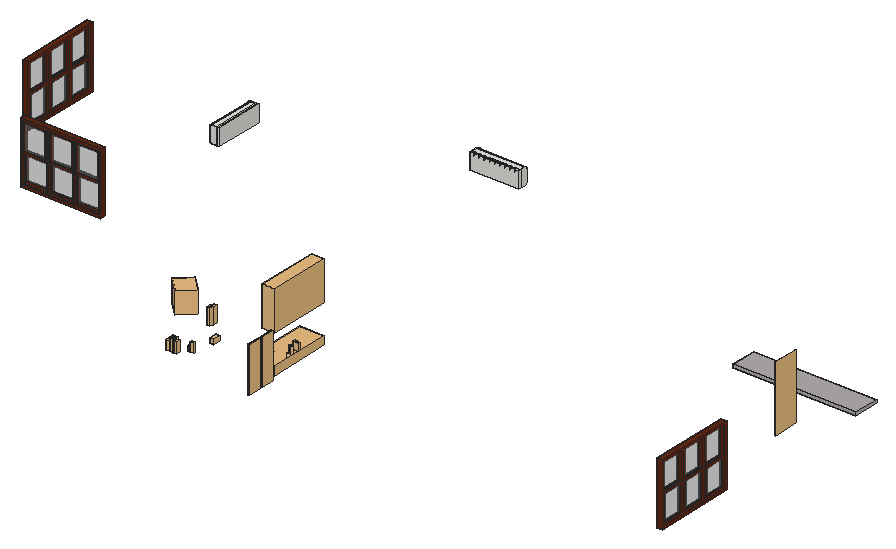
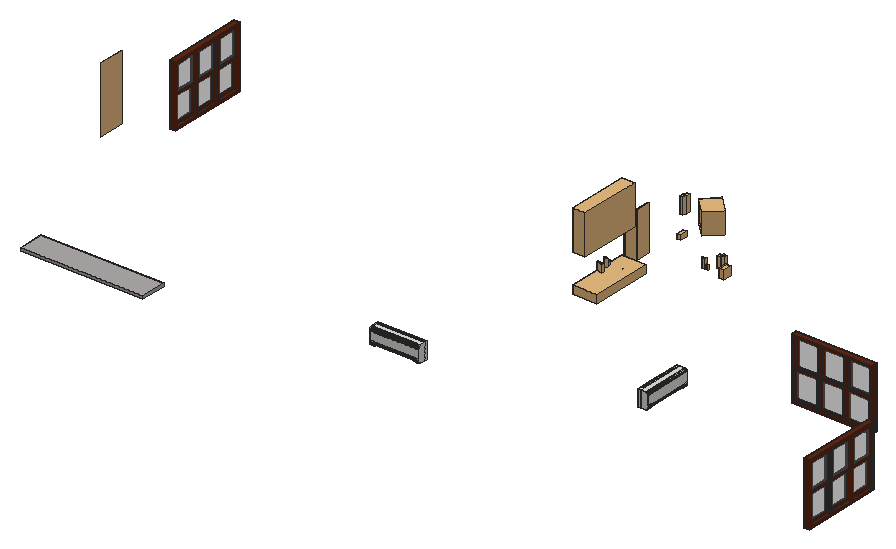
# SketchUp Ruby script. Lengths in inches.
U = 1.inch
M = Sketchup.active_model
def pt(a) = Geom::Point3d.new(a.map { |v| v * U })
def face(e, loops, mat)
  f = e.add_face(loops[0].map { |a| pt(a) })
  loops[1..].each { |l| e.add_face(l.map { |a| pt(a) }).erase! }
  f.material = f.back_material = mat if mat
  f
end
# faces: each face lists its corners as indices into pts; further lists are holes
def faces(e, pts, list, mat = nil) = list.each { |f| face(e, (f[0].is_a?(Array) ? f : [f]).map { |l| l.map { |i| pts[i] } }, mat) }
# xy, xz, yz: faces in a plane at the given z, y or x. An outline is a flat list of corners, or four numbers for a rectangle; further outlines are holes
def ring(l) = l.size == 4 ? [[l[0], l[1]], [l[2], l[1]], [l[2], l[3]], [l[0], l[3]]] : l.each_slice(2).to_a
def flat(e, list, mat, &to3) = list.each { |f| face(e, (f[0].is_a?(Array) ? f : [f]).map { |l| ring(l).map { |u, v| to3.(u, v) } }, mat) }
def xy(e, z, list, mat = nil) = flat(e, list, mat) { |x, y| [x, y, z] }
def xz(e, y, list, mat = nil) = flat(e, list, mat) { |x, z| [x, y, z] }
def yz(e, x, list, mat = nil) = flat(e, list, mat) { |y, z| [x, y, z] }
def lines(e, pts, list) = list.each { |a, b| e.add_line(pt(pts[a]), pt(pts[b])) }
# prism: a flat outline (further loops are holes) pulled along v
def prism(e, loops, v, mat = nil)
  f = face(e, loops, mat); d = Geom::Vector3d.new(v.map { |x| x * U })
  f.pushpull(f.normal.samedirection?(d) ? d.length : -d.length)
end
def box(e, o, s, mat = nil) = prism(e, [[o, [o[0] + s[0], o[1], o[2]], [o[0] + s[0], o[1] + s[1], o[2]], [o[0], o[1] + s[1], o[2]]]], [0, 0, s[2]], mat)
def at(x, y, z, deg = 0) = Geom::Transformation.translation(pt([x, y, z])) * Geom::Transformation.rotation(ORIGIN, Z_AXIS, deg.degrees)
def axes(o, x, y, z) = Geom::Transformation.new([*x, 0, *y, 0, *z, 0, *pt(o).to_a, 1])
def part(name) = M.definitions.add(name)
# library, detail: a bought-in or finely detailed component or shape, given as its bounding box
def library(name, o, s) = part(name).tap { |d| box(d.entities, o, s) }
def detail(e, o, s) = box(e.add_group.entities, o, s)
def put(e, d, t, mat = nil) = e.add_instance(d, t).tap { |i| i.material = mat if mat }
def group(e, t, mat = nil) = e.add_group.tap { |g| g.transformation = t; g.material = mat if mat }.entities
root = M.entities
M.materials.add("[0084_MediumTurquoise]").color = [178, 172, 172]
M.materials.add("[Color_004]").color = [142, 142, 142]
M.materials.add("[Color_005]").color = [114, 114, 114]
M.materials.add("[Color_007]").color = [58, 58, 58]
M.materials.add("[Color_B17]").color = [102, 40, 20]
M.materials.add("[Color_C12]").color = [153, 91, 30]
M.materials.add("[Translucent_Glass_Gray]").color = [128, 128, 128]
M.materials["[Translucent_Glass_Gray]"].alpha = 0.5
c1 = library("Group\#168",[0,0,0],[3.19,4.75,5.75])
c2 = library("Group\#184",[0,0,0],[13.47,43.07,1.47])
c3 = library("ear swab",[42.94,49.125,-0.01],[11.74,6.52,7.19])
c4 = library("Group\#182",[-0.16,-0.23,0],[24.67,28.96,29.58])
c5 = library("Group\#176",[0,0,0],[6.09,14.19,2.01])
c6 = library("Group\#177",[0,0,0],[5.65,13.74,2.92])
c7 = library("Group\#180",[0,0,0],[21.92,21.92,23.47])
c8 = library("Group\#181",[0,0,0],[23.26,37.79,80.08])
c9 = part("Framed panel")
g1 = group(c9.entities,at(0,0,0))
prism(g1,[[[0,22.64,0],[21.26,22.64,0],[21.26,0,0],[0,0,0]],[[1.57,1.57,0],[19.69,1.57,0],[19.69,21.0625,0],[1.57,21.0625,0]]],[0,0,1.57],"[Color_B17]")
g2 = group(c9.entities,at(1.57,1.57,1.02))
xy(g2,0,[[0,0,18.11,19.49]],"[Translucent_Glass_Gray]")
c10 = part("Group\#25")
put(c10.entities,c9,at(0,21.0625,1.57))
put(c10.entities,c9,at(0,0,0))
c11 = part("Group\#47")
g3 = group(c11.entities,at(0,0,0))
prism(g3,[[[70.87,0,0],[0,0,0],[0,47.24,0],[70.87,47.24,0]],[[47.83,1.77,0],[69.09,1.77,0],[69.09,45.47,0],[47.83,45.47,0]],[[46.0625,45.47,0],[24.8,45.47,0],[24.8,1.77,0],[46.0625,1.77,0]],[[1.77,1.77,0],[23.03,1.77,0],[23.03,45.47,0],[1.77,45.47,0]]],[0,0,4.33],"[Color_B17]")
put(c11.entities,c10,at(1.77,1.77,0.59))
put(c11.entities,c10,at(24.8,1.77,0.59))
put(c11.entities,c10,at(47.83,1.77,0.59))
c12 = part("Group\#165")
xy(c12.entities,0,[[3.14,0.77,2.7,0.83,2.28,1,1.93,1.27,1.65,1.63,1.48,2.04,4.8,2.93,4.86,2.49,4.8,2.04,4.63,1.63,4.36,1.27,4,1,3.59,0.83],[24.03,0.77,23.59,0.83,23.17,1,22.81,1.27,22.54,1.63,25.25,3.7,25.52,3.35,25.69,2.93,25.75,2.49,25.69,2.04,25.52,1.63,25.25,1.27,24.89,1,24.48,0.83],[22.54,1.63,22.37,2.04,22.3125,2.49,22.37,2.93,22.54,3.35,22.81,3.7,23.17,3.98,23.59,4.15,24.03,4.21,24.48,4.15,24.89,3.98,25.25,3.7],[1.48,2.04,1.42,2.49,1.48,2.93,1.65,3.35,1.93,3.7,2.28,3.98,2.7,4.15,3.14,4.21,3.59,4.15,4,3.98,4.36,3.7,4.63,3.35,4.8,2.93]],"[Color_005]")
xy(c12.entities,2.2,[[3.14,0.77,3.59,0.83,4,1,4.36,1.27,4.63,1.63,4.8,2.04,4.86,2.49,4.8,2.93,4.63,3.35,4.36,3.7,4,3.98,3.59,4.15,3.14,4.21,2.7,4.15,2.28,3.98,1.93,3.7,1.65,3.35,1.48,2.93,1.42,2.49,1.48,2.04,1.65,1.63,1.93,1.27,2.28,1,2.7,0.83],[24.03,0.77,24.48,0.83,24.89,1,25.25,1.27,25.52,1.63,25.69,2.04,25.75,2.49,25.69,2.93,25.52,3.35,25.25,3.7,24.89,3.98,24.48,4.15,24.03,4.21,23.59,4.15,23.17,3.98,22.81,3.7,22.54,3.35,22.37,2.93,22.3125,2.49,22.37,2.04,22.54,1.63,22.81,1.27,23.17,1,23.59,0.83]])
p = [[2.28,1,0],[2.7,0.83,0],[2.7,0.83,2.2],[2.28,1,2.2],[3.14,0.77,0],[3.14,0.77,2.2],
  [3.59,0.83,0],[3.59,0.83,2.2],[4,1,0],[4,1,2.2],[23.17,1,0],[23.59,0.83,0],
  [23.59,0.83,2.2],[23.17,1,2.2],[24.03,0.77,0],[24.03,0.77,2.2],[24.48,0.83,0],[24.48,0.83,2.2],
  [24.89,1,0],[24.89,1,2.2],[1.93,1.27,0],[1.93,1.27,2.2],[4.36,1.27,0],[4.36,1.27,2.2],
  [22.81,1.27,0],[22.81,1.27,2.2],[25.25,1.27,0],[25.25,1.27,2.2],[1.65,1.63,0],[1.65,1.63,2.2],
  [4.63,1.63,0],[4.63,1.63,2.2],[22.54,1.63,0],[22.54,1.63,2.2],[25.52,1.63,0],[25.52,1.63,2.2],
  [1.48,2.04,0],[1.48,2.04,2.2],[4.8,2.04,0],[4.8,2.04,2.2],[22.37,2.04,0],[22.37,2.04,2.2],
  [25.69,2.04,0],[25.69,2.04,2.2],[1.42,2.49,0],[1.42,2.49,2.2],[4.86,2.49,0],[4.86,2.49,2.2],
  [22.3125,2.49,0],[22.3125,2.49,2.2],[25.75,2.49,0],[25.75,2.49,2.2],[1.48,2.93,0],[1.48,2.93,2.2],
  [4.8,2.93,0],[4.8,2.93,2.2],[22.37,2.93,0],[22.37,2.93,2.2],[25.69,2.93,0],[25.69,2.93,2.2],
  [1.65,3.35,0],[1.65,3.35,2.2],[4.63,3.35,0],[4.63,3.35,2.2],[22.54,3.35,0],[22.54,3.35,2.2],
  [25.52,3.35,0],[25.52,3.35,2.2],[1.93,3.7,0],[1.93,3.7,2.2],[4.36,3.7,0],[4.36,3.7,2.2],
  [22.81,3.7,0],[22.81,3.7,2.2],[25.25,3.7,0],[25.25,3.7,2.2],[2.28,3.98,0],[2.28,3.98,2.2],
  [4,3.98,0],[4,3.98,2.2],[23.17,3.98,0],[23.17,3.98,2.2],[24.89,3.98,0],[24.89,3.98,2.2],
  [2.7,4.15,0],[2.7,4.15,2.2],[3.59,4.15,0],[3.59,4.15,2.2],[23.59,4.15,0],[23.59,4.15,2.2],
  [24.48,4.15,0],[24.48,4.15,2.2],[3.14,4.21,0],[3.14,4.21,2.2],[24.03,4.21,0],[24.03,4.21,2.2]]
faces(c12.entities,p,[[0,1,2,3],[1,4,5,2],[4,6,7,5],[6,8,9,7],[10,11,12,13],[11,14,15,12],[14,16,17,15],[16,18,19,17],
  [20,0,3,21],[8,22,23,9],[24,10,13,25],[18,26,27,19],[28,20,21,29],[22,30,31,23],[32,24,25,33],[26,34,35,27],
  [36,28,29,37],[30,38,39,31],[40,32,33,41],[34,42,43,35],[44,36,37,45],[38,46,47,39],[48,40,41,49],[42,50,51,43],
  [52,44,45,53],[46,54,55,47],[56,48,49,57],[50,58,59,51],[60,52,53,61],[54,62,63,55],[64,56,57,65],[58,66,67,59],
  [68,60,61,69],[62,70,71,63],[72,64,65,73],[66,74,75,67],[76,68,69,77],[70,78,79,71],[80,72,73,81],[74,82,83,75],
  [84,76,77,85],[78,86,87,79],[88,80,81,89],[82,90,91,83],[92,84,85,93],[86,92,93,87],[94,88,89,95],[90,94,95,91]],"[Color_005]")
g4 = group(c12.entities,at(0,0,1.83),"[Color_005]")
box(g4,[0,0,0],[27.7,4.93,1.59])
c13 = library("Group\#189",[-0.38,0,0],[4.27,10.97,14.2])
c14 = library("Group\#188",[0,0,0],[19.07,47.48,6.54])
c15 = library("Group\#186",[0,0,0],[47.48,30.74,9.84])
c16 = library("Group\#224",[0,202.4,-2.65],[190.5,180.61,2.65])
c17 = library("Group\#73",[-80.34,-149.03,-93.91],[1.18,2.79,3])
c18 = library("Group\#74",[-80.34,-139.83,-93.89],[1.18,2.84,2.98])
c19 = library("Group\#63",[-80.46,-65.36,-92.6],[1.38,3.58,3.59])
p = [[1618.6875,177.45,34.42],[1618.76,177.12,35.41],[1618.76,177.1,35.41]]
faces(root,p,[[0,1,2]])
g5 = group(root,at(1599.51,140.375,64.56))
detail(g5,[-0.37,-2.82,0],[2.54,2.53,12.33])
g6 = group(root,at(1571.03,141.11,35.64))
detail(g6,[-1.27,-3.0625,0],[2.54,2.53,9.2])
g7 = group(root,at(1575.59,140.06,35.64))
detail(g7,[-3,-1.73,0],[2.54,2.53,8.61])
g8 = group(root,at(1602.34,143.09,64.56))
detail(g8,[-2.7,-2.7,0],[2.7,2.7,12.33])
put(root,c1,axes([1568.21,147.6,33.83],[-1.2,0,0],[0,-1.416,0],[0,0,1.2]))
put(root,c2,axes([1630.57,149.66,26.11],[0,-0.77,0],[0,0,0.80496],[-1,0,0]))
put(root,c3,axes([1625.67,120.32,49.79],[0,0.5,0],[-0.5,0,0],[0,0,0.5]))
put(root,c4,axes([1574.96,155.51,64.56],[-0.39598,-0.39598,0],[0.39598,-0.39598,0],[0,0,0.56]))
put(root,c5,axes([1579.89,146.53,35.64],[0.5,0,0],[0,0,0.5],[0,-0.5,0]))
put(root,c6,axes([1578.03,146.54,35.64],[0.25,0,0],[0,0,0.25],[0,-0.25,0]))
put(root,c2,axes([1630.57,162.07,26.11],[0,-0.77,0],[0,0,0.80496],[-1,0,0]))
put(root,c7,axes([1628.03,178.13,35.52],[0.06654,-0.06654,0],[0.06654,0.06654,0],[0,0,0.09411]))
put(root,c8,axes([1628.3125,182.5,35.43],[-0.03711,-0.06428,0],[0.06428,-0.03711,0],[0,0,0.07422]))
put(root,c11,axes([1939.4375,213.95,36],[0,-0.87489,0],[0,0,1.016],[-1,0,0]))
put(root,c12,axes([1618.76,192.77,24.02],[0,-0.3762,0],[0,0,0.25582],[-0.3762,0,0]))
put(root,c13,axes([1626.17,188.26,35.43],[0,-0.39,0],[0.39,0,0],[0,0,0.39]),"[Color_005]")
put(root,c14,at(1630.57,211.45,28.89,-180))
put(root,c15,axes([1630.57,211.45,58.17],[0,-1,0],[0,0,1],[-1,0,0]))
put(root,c11,axes([1373.72,243.48,36],[0.87489,0,0],[0,0,1.016],[0,-1,0]))
put(root,c16,axes([1942.8125,275.9,0],[0,-0.10244,-0.00004],[0,-0.00011,0.28043],[-0.22,0,0]))
g9 = group(root,at(1470.58,328.97,79.75))
prism(g9,[[[-7.07,-15.5,-9.29],[-7.07,-15.45,-9.6],[-7.07,-15.52,-9.6],[-7.07,-15.57,-9.29]]],[0.1,0,0],"[Color_004]")
g10 = group(root,at(1470.58,328.97,79.75))
detail(g10,[-7.07,-15.51,-9.71],[0.1,0.08,0.08])
put(root,c17,axes([1470.58,328.97,79.75],[0.088,0,0],[0,0.10336,0],[0,0,0.10336]))
g11 = group(root,at(1470.58,328.97,79.75),"[Color_004]")
prism(g11,[[[-7.07,-15.07,-9.4],[-7.07,-14.96,-9.6],[-7.07,-14.92,-9.4],[-7.07,-14.85,-9.4],[-7.07,-14.91,-9.7],[-7.07,-14.98,-9.7],[-7.07,-15.15,-9.4]]],[0.1,0,0],"[Color_004]")
g12 = group(root,at(1470.58,328.97,79.75))
detail(g12,[-7.07,-14.86,-9.37],[0.1,0.08,0.08])
g13 = group(root,at(1470.58,328.97,79.75))
prism(g13,[[[-7.07,-14.79,-9.7],[-7.07,-14.84,-9.4],[-7.07,-14.77,-9.4],[-7.07,-14.72,-9.7]]],[0.1,0,0],"[Color_004]")
g14 = group(root,at(1470.58,328.97,79.75))
detail(g14,[-7.07,-14.73,-9.7],[0.1,0.25,0.41])
put(root,c18,axes([1470.58,328.97,79.75],[0.088,0,0],[0,0.10336,0],[0,0,0.10336]))
put(root,c19,axes([1470.57,328.97,79.75],[0.088,0,0],[0,0.10336,0],[0,0,0.10336]))
put(root,c11,axes([1334.35,357.95,36],[0,-0.87489,0],[0,0,1.016],[-1,0,0]))
g15 = group(root,at(1470.64,328.97,79.75))
xy(g15,-12.74,[[-1.73,-18.76,0,18.76]])
xy(g15,-2.26,[[-0.93,-15.67,-0.73,-11.93],[-0.64,-15.67,-0.43,-11.93],[-0.35,-15.67,-0.14,-11.93],[-0.93,-11.73,-0.73,-7.99],[-0.64,-11.73,-0.43,-7.99],
  [-0.35,-11.73,-0.14,-7.99],[-0.93,-7.79,-0.73,-4.04],[-0.64,-7.79,-0.43,-4.04],[-0.35,-7.79,-0.14,-4.04],[-0.93,-3.84,-0.73,-0.1],
  [-0.64,-3.84,-0.43,-0.1],[-0.35,-3.84,-0.14,-0.1],[-0.93,0.1,-0.73,3.84],[-0.64,0.1,-0.43,3.84],[-0.35,0.1,-0.14,3.84],
  [-0.93,4.04,-0.73,7.79],[-0.64,4.04,-0.43,7.79],[-0.35,4.04,-0.14,7.79],[-0.93,7.99,-0.73,11.73],[-0.64,7.99,-0.43,11.73],
  [-0.35,7.99,-0.14,11.73],[-0.93,11.93,-0.73,15.67],[-0.64,11.93,-0.43,15.67],[-0.35,11.93,-0.14,15.67]])
xy(g15,0,[[[-1.73,-18.76,0,18.76],[-0.93,4.04,-0.93,11.73,-0.73,11.73,-0.73,7.99,-0.93,7.99,-0.93,7.79,-0.73,7.79,-0.73,4.04],[-0.35,4.04,-0.35,7.79,-0.14,7.79,-0.14,7.99,-0.35,7.99,-0.35,11.73,-0.14,11.73,-0.14,4.04],[-0.64,11.93,-0.43,15.67],[-0.35,11.93,-0.14,15.67],[-0.93,11.93,-0.73,15.67],[-0.93,-15.67,-0.73,-11.93],[-0.35,-15.67,-0.14,-11.93],[-0.64,-15.67,-0.43,-11.93],[-0.64,4.04,-0.43,7.79],[-0.35,-7.79,-0.14,-4.04],[-0.64,-7.79,-0.43,-4.04],[-0.93,-7.79,-0.73,-4.04],[-0.64,7.99,-0.43,11.73],[-0.64,0.1,-0.43,3.84],[-0.35,0.1,-0.14,3.84],[-0.93,0.1,-0.73,3.84],[-0.35,-11.73,-0.14,-7.99],[-0.93,-11.73,-0.73,-7.99],[-0.93,-3.84,-0.73,-0.1],[-0.64,-3.84,-0.43,-0.1],[-0.35,-3.84,-0.14,-0.1],[-0.64,-11.73,-0.43,-7.99]]])
xz(g15,-18.76,[[-1.73,-12.74,0,0]])
xz(g15,-15.67,[[-0.93,-2.26,-0.73,0],[-0.64,-2.26,-0.43,0],[-0.35,-2.26,-0.14,0]])
xz(g15,-11.93,[[-0.93,-2.26,-0.73,0],[-0.64,-2.26,-0.43,0],[-0.35,-2.26,-0.14,0]])
xz(g15,-11.73,[[-0.93,-2.26,-0.73,0],[-0.64,-2.26,-0.43,0],[-0.35,-2.26,-0.14,0]])
xz(g15,-7.99,[[-0.93,-2.26,-0.73,0],[-0.64,-2.26,-0.43,0],[-0.35,-2.26,-0.14,0]])
xz(g15,-7.79,[[-0.93,-2.26,-0.73,0],[-0.64,-2.26,-0.43,0],[-0.35,-2.26,-0.14,0]])
xz(g15,-4.04,[[-0.93,-2.26,-0.73,0],[-0.64,-2.26,-0.43,0],[-0.35,-2.26,-0.14,0]])
xz(g15,-3.84,[[-0.93,-2.26,-0.73,0],[-0.64,-2.26,-0.43,0],[-0.35,-2.26,-0.14,0]])
xz(g15,-0.1,[[-0.93,-2.26,-0.73,0],[-0.64,-2.26,-0.43,0],[-0.35,-2.26,-0.14,0]])
xz(g15,0.1,[[-0.93,-2.26,-0.73,0],[-0.64,-2.26,-0.43,0],[-0.35,-2.26,-0.14,0]])
xz(g15,3.84,[[-0.93,-2.26,-0.73,0],[-0.64,-2.26,-0.43,0],[-0.35,-2.26,-0.14,0]])
xz(g15,4.04,[[-0.93,-2.26,-0.73,0],[-0.64,-2.26,-0.43,0],[-0.35,-2.26,-0.14,0]])
xz(g15,7.79,[[-0.93,-2.26,-0.73,0],[-0.64,-2.26,-0.43,0],[-0.35,-2.26,-0.14,0]])
xz(g15,7.99,[[-0.93,-2.26,-0.73,0],[-0.64,-2.26,-0.43,0],[-0.35,-2.26,-0.14,0]])
xz(g15,11.73,[[-0.93,-2.26,-0.73,0],[-0.64,-2.26,-0.43,0],[-0.35,-2.26,-0.14,0]])
xz(g15,11.93,[[-0.93,-2.26,-0.73,0],[-0.64,-2.26,-0.43,0],[-0.35,-2.26,-0.14,0]])
xz(g15,15.67,[[-0.93,-2.26,-0.73,0],[-0.64,-2.26,-0.43,0],[-0.35,-2.26,-0.14,0]])
xz(g15,18.76,[[-1.73,-12.74,0,0]])
yz(g15,-1.73,[[-18.76,-12.74,18.76,0]])
yz(g15,-0.93,[[-15.67,-2.26,-11.93,0],[-11.73,-2.26,-7.99,0],[-7.79,-2.26,-4.04,0],[-3.84,-2.26,-0.1,0],[0.1,-2.26,3.84,0],
  [4.04,-2.26,7.79,0],[7.99,-2.26,11.73,0],[11.93,-2.26,15.67,0]])
yz(g15,-0.73,[[-15.67,-2.26,-11.93,0],[-11.73,-2.26,-7.99,0],[-7.79,-2.26,-4.04,0],[-3.84,-2.26,-0.1,0],[0.1,-2.26,3.84,0],
  [4.04,-2.26,7.79,0],[7.99,-2.26,11.73,0],[11.93,-2.26,15.67,0]])
yz(g15,-0.64,[[-15.67,-2.26,-11.93,0],[-11.73,-2.26,-7.99,0],[-7.79,-2.26,-4.04,0],[-3.84,-2.26,-0.1,0],[0.1,-2.26,3.84,0],
  [4.04,-2.26,7.79,0],[7.99,-2.26,11.73,0],[11.93,-2.26,15.67,0]])
yz(g15,-0.43,[[-15.67,-2.26,-11.93,0],[-11.73,-2.26,-7.99,0],[-7.79,-2.26,-4.04,0],[-3.84,-2.26,-0.1,0],[0.1,-2.26,3.84,0],
  [4.04,-2.26,7.79,0],[7.99,-2.26,11.73,0],[11.93,-2.26,15.67,0]])
yz(g15,-0.35,[[-15.67,-2.26,-11.93,0],[-11.73,-2.26,-7.99,0],[-7.79,-2.26,-4.04,0],[-3.84,-2.26,-0.1,0],[0.1,-2.26,3.84,0],
  [4.04,-2.26,7.79,0],[7.99,-2.26,11.73,0],[11.93,-2.26,15.67,0]])
yz(g15,-0.14,[[-15.67,-2.26,-11.93,0],[-11.73,-2.26,-7.99,0],[-7.79,-2.26,-4.04,0],[-3.84,-2.26,-0.1,0],[0.1,-2.26,3.84,0],
  [4.04,-2.26,7.79,0],[7.99,-2.26,11.73,0],[11.93,-2.26,15.67,0]])
yz(g15,0,[[-18.76,-12.74,18.76,0]])
g16 = group(root,at(1470.64,328.97,79.75))
xy(g16,-12.74,[[-5.65,-18.76,-1.73,-15.875],[-5.65,15.875,-1.73,18.76]])
xy(g16,-9.91,[[-7.03,-15.875,-1.73,15.875]])
xy(g16,-9.7,[[-7.03,-3.48,-6.93,3.48]])
xy(g16,-9.07,[[-7.03,-3.48,-6.93,3.48]])
xy(g16,-8.96,[[-7.73,-18.76,-7.62,-15.875],[-7.62,-15.875,-7.03,15.875],[-7.73,15.875,-7.62,18.76]])
xy(g16,0,[[-5.65,-18.76,-1.73,18.76]])
xz(g16,-18.76,[[-5.65,-12.74,-1.73,-12.74,-1.73,0,-5.65,0,-5.65,-0.12,-5.96,-0.15,-6.26,-0.24,-6.54,-0.375,-6.81,-0.57,-7.04,-0.8,-7.24,-1.08,-7.41,-1.39,-7.53,-1.72,-7.6,-2.08,-7.62,-2.44,-7.62,-8.96,-7.73,-8.96,-7.73,-10.29,-7.7,-10.68,-7.625,-11.05,-7.5,-11.4,-7.33,-11.73,-7.12,-12.02,-6.87,-12.27,-6.59,-12.47,-6.29,-12.62,-5.97,-12.71]])
xz(g16,-15.875,[[-5.65,-12.74,-5.97,-12.71,-6.29,-12.62,-6.59,-12.47,-6.87,-12.27,-7.12,-12.02,-7.33,-11.73,-7.5,-11.4,-7.625,-11.05,-7.7,-10.68,-7.73,-10.29,-7.73,-8.96,-7.03,-8.96,-7.03,-9.91,-1.73,-9.91,-1.73,-12.74]])
xz(g16,-3.48,[[-7.03,-9.7,-6.93,-9.07]])
xz(g16,3.48,[[-7.03,-9.7,-6.93,-9.07]])
xz(g16,15.875,[[-5.65,-12.74,-1.73,-12.74,-1.73,-9.91,-7.03,-9.91,-7.03,-8.96,-7.73,-8.96,-7.73,-10.29,-7.7,-10.68,-7.625,-11.05,-7.5,-11.4,-7.33,-11.73,-7.12,-12.02,-6.87,-12.27,-6.59,-12.47,-6.29,-12.62,-5.97,-12.71]])
xz(g16,18.76,[[-5.65,-12.74,-5.97,-12.71,-6.29,-12.62,-6.59,-12.47,-6.87,-12.27,-7.12,-12.02,-7.33,-11.73,-7.5,-11.4,-7.625,-11.05,-7.7,-10.68,-7.73,-10.29,-7.73,-8.96,-7.62,-8.96,-7.62,-2.44,-7.6,-2.08,-7.53,-1.72,-7.41,-1.39,-7.24,-1.08,-7.04,-0.8,-6.81,-0.57,-6.54,-0.375,-6.26,-0.24,-5.96,-0.15,-5.65,-0.12,-5.65,0,-1.73,0,-1.73,-12.74]])
yz(g16,-7.73,[[-18.76,-10.29,-15.875,-8.96],[15.875,-10.29,18.76,-8.96]])
yz(g16,-7.62,[[-18.76,-8.96,18.76,-2.44]])
yz(g16,-7.03,[[[-15.875,-9.91,15.875,-8.96],[-3.48,-9.7,3.48,-9.07]]])
yz(g16,-6.93,[[-3.48,-9.7,3.48,-9.07]],"[Color_007]")
yz(g16,-5.65,[[-18.76,-0.12,18.76,0]])
yz(g16,-1.73,[[-18.76,-12.74,-15.875,-12.74,-15.875,-9.91,15.875,-9.91,15.875,-12.74,18.76,-12.74,18.76,0,-18.76,0]])
p = [[-6.29,-18.76,-12.62],[-6.29,-15.875,-12.62],[-5.97,-15.875,-12.71],[-5.97,-18.76,-12.71],[-5.65,-15.875,-12.74],[-5.65,-18.76,-12.74],
  [-6.29,15.875,-12.62],[-6.29,18.76,-12.62],[-5.97,18.76,-12.71],[-5.97,15.875,-12.71],[-5.65,18.76,-12.74],[-5.65,15.875,-12.74],
  [-6.59,-15.875,-12.47],[-6.59,-18.76,-12.47],[-6.59,15.875,-12.47],[-6.59,18.76,-12.47],[-6.87,-18.76,-12.27],[-6.87,-15.875,-12.27],
  [-6.87,15.875,-12.27],[-6.87,18.76,-12.27],[-7.12,-18.76,-12.02],[-7.12,-15.875,-12.02],[-7.12,15.875,-12.02],[-7.12,18.76,-12.02],
  [-7.33,-18.76,-11.73],[-7.33,-15.875,-11.73],[-7.33,15.875,-11.73],[-7.33,18.76,-11.73],[-7.5,-18.76,-11.4],[-7.5,-15.875,-11.4],
  [-7.5,15.875,-11.4],[-7.5,18.76,-11.4],[-7.625,-15.875,-11.05],[-7.625,-18.76,-11.05],[-7.625,15.875,-11.05],[-7.625,18.76,-11.05],
  [-7.7,-18.76,-10.68],[-7.7,-15.875,-10.68],[-7.7,15.875,-10.68],[-7.7,18.76,-10.68],[-7.73,-18.76,-10.29],[-7.73,-15.875,-10.29],
  [-7.73,15.875,-10.29],[-7.73,18.76,-10.29],[-7.62,18.76,-2.44],[-7.62,-18.76,-2.44],[-7.6,-18.76,-2.08],[-7.6,18.76,-2.08],
  [-7.53,-18.76,-1.72],[-7.53,18.76,-1.72],[-7.41,18.76,-1.39],[-7.41,-18.76,-1.39],[-7.24,-18.76,-1.08],[-7.24,18.76,-1.08],
  [-7.04,-18.76,-0.8],[-7.04,18.76,-0.8],[-6.81,-18.76,-0.57],[-6.81,18.76,-0.57],[-6.54,-18.76,-0.375],[-6.54,18.76,-0.375],
  [-6.26,18.76,-0.24],[-6.26,-18.76,-0.24],[-5.96,-18.76,-0.15],[-5.96,18.76,-0.15],[-5.65,-18.76,-0.12],[-5.65,18.76,-0.12]]
faces(g16,p,[[0,1,2,3],[4,5,3,2],[6,7,8,9],[10,11,9,8],[12,1,0,13],[6,14,15,7],[12,13,16,17],[15,14,18,19],
  [20,21,17,16],[22,23,19,18],[21,20,24,25],[23,22,26,27],[28,29,25,24],[30,31,27,26],[32,29,28,33],[30,34,35,31],
  [32,33,36,37],[35,34,38,39],[40,41,37,36],[42,43,39,38],[44,45,46,47],[48,49,47,46],[50,49,48,51],[50,51,52,53],
  [54,55,53,52],[55,54,56,57],[58,59,57,56],[60,59,58,61],[60,61,62,63],[64,65,63,62]])
g17 = group(root,at(1470.64,328.97,79.75))
prism(g17,[[[-7.73,18.74,-8.96],[-7.73,18.74,-2.44],[-7.7,18.74,-2.06],[-7.625,18.74,-1.6875],[-7.5,18.74,-1.33],[-7.33,18.74,-1.01],[-7.12,18.74,-0.72],[-6.87,18.74,-0.47],[-6.59,18.74,-0.27],[-6.29,18.74,-0.12],[-5.97,18.74,-0.03],[-5.65,18.74,0],[-5.65,18.74,-0.12],[-5.96,18.74,-0.15],[-6.26,18.74,-0.24],[-6.54,18.74,-0.375],[-6.81,18.74,-0.57],[-7.04,18.74,-0.8],[-7.24,18.74,-1.08],[-7.41,18.74,-1.39],[-7.53,18.74,-1.72],[-7.6,18.74,-2.08],[-7.62,18.74,-2.44],[-7.62,18.74,-8.96]]],[0,-37.47,0])
g18 = group(root,at(1470.64,328.97,79.75))
xy(g18,-12.375,[[-5.58,-15.875,-3.67,15.875]])
xy(g18,-10.42,[[-7.25,-15.875,-7,-9.1],[-7.25,-8.85,-7,4.71],[-7.25,4.95,-7,15.875]])
xy(g18,-9.91,[[-7,-15.875,-3.67,-15.875,-3.67,15.875,-7,15.875,-7,4.95,-7.25,4.95,-7.25,4.71,-7,4.71,-7,-8.85,-7.25,-8.85,-7.25,-9.1,-7,-9.1]])
xz(g18,-15.875,[[-5.58,-12.375,-3.67,-12.375,-3.67,-9.91,-7,-9.91,-7,-10.42,-7.25,-10.42,-7.24,-10.46,-7.23,-10.73,-7.17,-11.02,-7.07,-11.31,-6.93,-11.57,-6.76,-11.8,-6.5625,-12,-6.34,-12.16,-6.1,-12.28,-5.84,-12.35]])
xz(g18,-9.1,[[-7.25,-10.42,-7,-9.91]])
xz(g18,-8.85,[[-7.25,-10.42,-7,-9.91]])
xz(g18,4.71,[[-7.25,-10.42,-7,-9.91]])
xz(g18,4.95,[[-7.25,-10.42,-7,-9.91]])
xz(g18,15.875,[[-5.58,-12.375,-5.84,-12.35,-6.1,-12.28,-6.34,-12.16,-6.5625,-12,-6.76,-11.8,-6.93,-11.57,-7.07,-11.31,-7.17,-11.02,-7.23,-10.73,-7.24,-10.46,-7.25,-10.42,-7,-10.42,-7,-9.91,-3.67,-9.91,-3.67,-12.375]])
yz(g18,-7.25,[[-9.1,-10.42,-8.85,-9.91],[4.71,-10.42,4.95,-9.91]])
yz(g18,-7,[[-15.875,-10.42,-9.1,-9.91],[-8.85,-10.42,4.71,-9.91],[4.95,-10.42,15.875,-9.91]],"[Color_007]")
yz(g18,-3.67,[[-15.875,-12.375,15.875,-9.91]])
p = [[-5.58,15.875,-12.375],[-5.58,-15.875,-12.375],[-5.84,-15.875,-12.35],[-5.84,15.875,-12.35],[-6.34,15.875,-12.16],[-6.1,15.875,-12.28],
  [-6.1,-15.875,-12.28],[-6.34,-15.875,-12.16],[-6.5625,-15.875,-12],[-6.5625,15.875,-12],[-6.76,-15.875,-11.8],[-6.76,15.875,-11.8],
  [-6.93,-15.875,-11.57],[-6.93,15.875,-11.57],[-7.07,-15.875,-11.31],[-7.07,15.875,-11.31],[-7.17,15.875,-11.02],[-7.17,-15.875,-11.02],
  [-7.23,-15.875,-10.73],[-7.23,15.875,-10.73],[-7.24,-15.875,-10.46],[-7.24,-9.1,-10.46],[-7.24,-8.85,-10.46],[-7.24,4.71,-10.46],
  [-7.24,4.95,-10.46],[-7.24,15.875,-10.46],[-7.25,15.875,-10.42],[-7.25,-15.875,-10.42],[-7.25,-9.1,-10.42],[-7.25,-8.85,-10.42],
  [-7.25,4.71,-10.42],[-7.25,4.95,-10.42]]
faces(g18,p,[[0,1,2,3],[4,5,6,7],[6,5,3,2],[4,7,8,9],[10,11,9,8],[11,10,12,13],[14,15,13,12],[16,15,14,17],
  [16,17,18,19],[18,20,21,22,23,24,25,19]])
faces(g18,p,[[26,25,24,23,22,21,20,27,28,29,30,31]],"[Color_C12]")
g19 = group(root,at(1834.62,351.14,23.97),"[0084_MediumTurquoise]")
box(g19,[0,0,0],[94.73,19.71,2.36],"[0084_MediumTurquoise]")
g20 = group(root,at(1625.625,381.93,79.75))
xy(g20,-12.74,[[-18.76,0,18.76,1.73]])
xy(g20,-2.26,[[-15.67,0.14,-11.93,0.35],[-11.73,0.14,-7.99,0.35],[-7.79,0.14,-4.04,0.35],[-3.84,0.14,-0.1,0.35],[0.1,0.14,3.84,0.35],
  [4.04,0.14,7.79,0.35],[7.99,0.14,11.73,0.35],[11.93,0.14,15.67,0.35],[-15.67,0.43,-11.93,0.64],[-11.73,0.43,-7.99,0.64],
  [-7.79,0.43,-4.04,0.64],[-3.84,0.43,-0.1,0.64],[0.1,0.43,3.84,0.64],[4.04,0.43,7.79,0.64],[7.99,0.43,11.73,0.64],
  [11.93,0.43,15.67,0.64],[-15.67,0.73,-11.93,0.93],[-11.73,0.73,-7.99,0.93],[-7.79,0.73,-4.04,0.93],[-3.84,0.73,-0.1,0.93],
  [0.1,0.73,3.84,0.93],[4.04,0.73,7.79,0.93],[7.99,0.73,11.73,0.93],[11.93,0.73,15.67,0.93]])
xy(g20,0,[[[-18.76,0,18.76,1.73],[4.04,0.73,4.04,0.93,11.73,0.93,11.73,0.73,7.99,0.73,7.99,0.93,7.79,0.93,7.79,0.73],[4.04,0.14,4.04,0.35,7.79,0.35,7.79,0.14,7.99,0.14,7.99,0.35,11.73,0.35,11.73,0.14],[11.93,0.43,15.67,0.64],[11.93,0.14,15.67,0.35],[11.93,0.73,15.67,0.93],[-15.67,0.73,-11.93,0.93],[-15.67,0.14,-11.93,0.35],[-15.67,0.43,-11.93,0.64],[4.04,0.43,7.79,0.64],[-7.79,0.14,-4.04,0.35],[-7.79,0.43,-4.04,0.64],[-7.79,0.73,-4.04,0.93],[7.99,0.43,11.73,0.64],[0.1,0.43,3.84,0.64],[0.1,0.14,3.84,0.35],[0.1,0.73,3.84,0.93],[-11.73,0.14,-7.99,0.35],[-11.73,0.73,-7.99,0.93],[-3.84,0.73,-0.1,0.93],[-3.84,0.43,-0.1,0.64],[-3.84,0.14,-0.1,0.35],[-11.73,0.43,-7.99,0.64]]])
xz(g20,0,[[-18.76,-12.74,18.76,0]])
xz(g20,0.14,[[-15.67,-2.26,-11.93,0],[-11.73,-2.26,-7.99,0],[-7.79,-2.26,-4.04,0],[-3.84,-2.26,-0.1,0],[0.1,-2.26,3.84,0],
  [4.04,-2.26,7.79,0],[7.99,-2.26,11.73,0],[11.93,-2.26,15.67,0]])
xz(g20,0.35,[[-15.67,-2.26,-11.93,0],[-11.73,-2.26,-7.99,0],[-7.79,-2.26,-4.04,0],[-3.84,-2.26,-0.1,0],[0.1,-2.26,3.84,0],
  [4.04,-2.26,7.79,0],[7.99,-2.26,11.73,0],[11.93,-2.26,15.67,0]])
xz(g20,0.43,[[-15.67,-2.26,-11.93,0],[-11.73,-2.26,-7.99,0],[-7.79,-2.26,-4.04,0],[-3.84,-2.26,-0.1,0],[0.1,-2.26,3.84,0],
  [4.04,-2.26,7.79,0],[7.99,-2.26,11.73,0],[11.93,-2.26,15.67,0]])
xz(g20,0.64,[[-15.67,-2.26,-11.93,0],[-11.73,-2.26,-7.99,0],[-7.79,-2.26,-4.04,0],[-3.84,-2.26,-0.1,0],[0.1,-2.26,3.84,0],
  [4.04,-2.26,7.79,0],[7.99,-2.26,11.73,0],[11.93,-2.26,15.67,0]])
xz(g20,0.73,[[-15.67,-2.26,-11.93,0],[-11.73,-2.26,-7.99,0],[-7.79,-2.26,-4.04,0],[-3.84,-2.26,-0.1,0],[0.1,-2.26,3.84,0],
  [4.04,-2.26,7.79,0],[7.99,-2.26,11.73,0],[11.93,-2.26,15.67,0]])
xz(g20,0.93,[[-15.67,-2.26,-11.93,0],[-11.73,-2.26,-7.99,0],[-7.79,-2.26,-4.04,0],[-3.84,-2.26,-0.1,0],[0.1,-2.26,3.84,0],
  [4.04,-2.26,7.79,0],[7.99,-2.26,11.73,0],[11.93,-2.26,15.67,0]])
xz(g20,1.73,[[-18.76,-12.74,18.76,0]])
yz(g20,-18.76,[[0,-12.74,1.73,0]])
yz(g20,-15.67,[[0.14,-2.26,0.35,0],[0.43,-2.26,0.64,0],[0.73,-2.26,0.93,0]])
yz(g20,-11.93,[[0.14,-2.26,0.35,0],[0.43,-2.26,0.64,0],[0.73,-2.26,0.93,0]])
yz(g20,-11.73,[[0.14,-2.26,0.35,0],[0.43,-2.26,0.64,0],[0.73,-2.26,0.93,0]])
yz(g20,-7.99,[[0.14,-2.26,0.35,0],[0.43,-2.26,0.64,0],[0.73,-2.26,0.93,0]])
yz(g20,-7.79,[[0.14,-2.26,0.35,0],[0.43,-2.26,0.64,0],[0.73,-2.26,0.93,0]])
yz(g20,-4.04,[[0.14,-2.26,0.35,0],[0.43,-2.26,0.64,0],[0.73,-2.26,0.93,0]])
yz(g20,-3.84,[[0.14,-2.26,0.35,0],[0.43,-2.26,0.64,0],[0.73,-2.26,0.93,0]])
yz(g20,-0.1,[[0.14,-2.26,0.35,0],[0.43,-2.26,0.64,0],[0.73,-2.26,0.93,0]])
yz(g20,0.1,[[0.14,-2.26,0.35,0],[0.43,-2.26,0.64,0],[0.73,-2.26,0.93,0]])
yz(g20,3.84,[[0.14,-2.26,0.35,0],[0.43,-2.26,0.64,0],[0.73,-2.26,0.93,0]])
yz(g20,4.04,[[0.14,-2.26,0.35,0],[0.43,-2.26,0.64,0],[0.73,-2.26,0.93,0]])
yz(g20,7.79,[[0.14,-2.26,0.35,0],[0.43,-2.26,0.64,0],[0.73,-2.26,0.93,0]])
yz(g20,7.99,[[0.14,-2.26,0.35,0],[0.43,-2.26,0.64,0],[0.73,-2.26,0.93,0]])
yz(g20,11.73,[[0.14,-2.26,0.35,0],[0.43,-2.26,0.64,0],[0.73,-2.26,0.93,0]])
yz(g20,11.93,[[0.14,-2.26,0.35,0],[0.43,-2.26,0.64,0],[0.73,-2.26,0.93,0]])
yz(g20,15.67,[[0.14,-2.26,0.35,0],[0.43,-2.26,0.64,0],[0.73,-2.26,0.93,0]])
yz(g20,18.76,[[0,-12.74,1.73,0]])
g21 = group(root,at(1625.625,381.93,79.75))
xy(g21,-12.74,[[-18.76,1.73,-15.875,5.65],[15.875,1.73,18.76,5.65]])
xy(g21,-9.91,[[-15.875,1.73,15.875,7.03]])
xy(g21,-9.7,[[-3.48,6.93,3.48,7.03]])
xy(g21,-9.07,[[-3.48,6.93,3.48,7.03]])
xy(g21,-8.96,[[-15.875,7.03,15.875,7.62],[-18.76,7.62,-15.875,7.73],[15.875,7.62,18.76,7.73]])
xy(g21,0,[[-18.76,1.73,18.76,5.65]])
xz(g21,1.73,[[-18.76,-12.74,-15.875,-12.74,-15.875,-9.91,15.875,-9.91,15.875,-12.74,18.76,-12.74,18.76,0,-18.76,0]])
xz(g21,5.65,[[-18.76,-0.12,18.76,0]])
xz(g21,6.93,[[-3.48,-9.7,3.48,-9.07]],"[Color_007]")
xz(g21,7.03,[[[-15.875,-9.91,15.875,-8.96],[-3.48,-9.7,3.48,-9.07]]])
xz(g21,7.62,[[-18.76,-8.96,18.76,-2.44]])
xz(g21,7.73,[[-18.76,-10.29,-15.875,-8.96],[15.875,-10.29,18.76,-8.96]])
yz(g21,-18.76,[[1.73,-12.74,1.73,0,5.65,0,5.65,-0.12,5.96,-0.15,6.26,-0.24,6.54,-0.375,6.81,-0.57,7.04,-0.8,7.24,-1.08,7.41,-1.39,7.53,-1.72,7.6,-2.08,7.62,-2.44,7.62,-8.96,7.73,-8.96,7.73,-10.29,7.7,-10.68,7.625,-11.05,7.5,-11.4,7.33,-11.73,7.12,-12.02,6.87,-12.27,6.59,-12.47,6.29,-12.62,5.97,-12.71,5.65,-12.74]])
yz(g21,-15.875,[[1.73,-12.74,5.65,-12.74,5.97,-12.71,6.29,-12.62,6.59,-12.47,6.87,-12.27,7.12,-12.02,7.33,-11.73,7.5,-11.4,7.625,-11.05,7.7,-10.68,7.73,-10.29,7.73,-8.96,7.03,-8.96,7.03,-9.91,1.73,-9.91]])
yz(g21,-3.48,[[6.93,-9.7,7.03,-9.07]])
yz(g21,3.48,[[6.93,-9.7,7.03,-9.07]])
yz(g21,15.875,[[1.73,-12.74,1.73,-9.91,7.03,-9.91,7.03,-8.96,7.73,-8.96,7.73,-10.29,7.7,-10.68,7.625,-11.05,7.5,-11.4,7.33,-11.73,7.12,-12.02,6.87,-12.27,6.59,-12.47,6.29,-12.62,5.97,-12.71,5.65,-12.74]])
yz(g21,18.76,[[1.73,-12.74,5.65,-12.74,5.97,-12.71,6.29,-12.62,6.59,-12.47,6.87,-12.27,7.12,-12.02,7.33,-11.73,7.5,-11.4,7.625,-11.05,7.7,-10.68,7.73,-10.29,7.73,-8.96,7.62,-8.96,7.62,-2.44,7.6,-2.08,7.53,-1.72,7.41,-1.39,7.24,-1.08,7.04,-0.8,6.81,-0.57,6.54,-0.375,6.26,-0.24,5.96,-0.15,5.65,-0.12,5.65,0,1.73,0]])
p = [[-15.875,5.65,-12.74],[-18.76,5.65,-12.74],[-18.76,5.97,-12.71],[-15.875,5.97,-12.71],[18.76,5.65,-12.74],[15.875,5.65,-12.74],
  [15.875,5.97,-12.71],[18.76,5.97,-12.71],[-18.76,6.29,-12.62],[-15.875,6.29,-12.62],[15.875,6.29,-12.62],[18.76,6.29,-12.62],
  [-15.875,6.59,-12.47],[-18.76,6.59,-12.47],[15.875,6.59,-12.47],[18.76,6.59,-12.47],[-18.76,6.87,-12.27],[-15.875,6.87,-12.27],
  [15.875,6.87,-12.27],[18.76,6.87,-12.27],[-18.76,7.12,-12.02],[-15.875,7.12,-12.02],[15.875,7.12,-12.02],[18.76,7.12,-12.02],
  [-18.76,7.33,-11.73],[-15.875,7.33,-11.73],[15.875,7.33,-11.73],[18.76,7.33,-11.73],[-18.76,7.5,-11.4],[-15.875,7.5,-11.4],
  [15.875,7.5,-11.4],[18.76,7.5,-11.4],[-15.875,7.625,-11.05],[-18.76,7.625,-11.05],[15.875,7.625,-11.05],[18.76,7.625,-11.05],
  [-18.76,7.7,-10.68],[-15.875,7.7,-10.68],[15.875,7.7,-10.68],[18.76,7.7,-10.68],[-18.76,7.73,-10.29],[-15.875,7.73,-10.29],
  [15.875,7.73,-10.29],[18.76,7.73,-10.29],[18.76,7.62,-2.44],[-18.76,7.62,-2.44],[-18.76,7.6,-2.08],[18.76,7.6,-2.08],
  [-18.76,7.53,-1.72],[18.76,7.53,-1.72],[18.76,7.41,-1.39],[-18.76,7.41,-1.39],[-18.76,7.24,-1.08],[18.76,7.24,-1.08],
  [-18.76,7.04,-0.8],[18.76,7.04,-0.8],[-18.76,6.81,-0.57],[18.76,6.81,-0.57],[-18.76,6.54,-0.375],[18.76,6.54,-0.375],
  [18.76,6.26,-0.24],[-18.76,6.26,-0.24],[-18.76,5.65,-0.12],[18.76,5.65,-0.12],[18.76,5.96,-0.15],[-18.76,5.96,-0.15]]
faces(g21,p,[[0,1,2,3],[4,5,6,7],[8,9,3,2],[10,11,7,6],[12,9,8,13],[10,14,15,11],[12,13,16,17],[15,14,18,19],
  [20,21,17,16],[22,23,19,18],[21,20,24,25],[23,22,26,27],[28,29,25,24],[30,31,27,26],[32,29,28,33],[30,34,35,31],
  [32,33,36,37],[35,34,38,39],[40,41,37,36],[42,43,39,38],[44,45,46,47],[48,49,47,46],[50,49,48,51],[50,51,52,53],
  [54,55,53,52],[55,54,56,57],[58,59,57,56],[60,59,58,61],[62,63,64,65],[60,61,65,64]])
g22 = group(root,at(1625.625,381.93,79.75))
xy(g22,-12.375,[[-15.875,3.67,15.875,5.58]])
xy(g22,-10.42,[[-15.875,7,-9.1,7.25],[-8.85,7,4.71,7.25],[4.95,7,15.875,7.25]])
xy(g22,-9.91,[[-15.875,3.67,15.875,3.67,15.875,7,4.95,7,4.95,7.25,4.71,7.25,4.71,7,-8.85,7,-8.85,7.25,-9.1,7.25,-9.1,7,-15.875,7]])
xz(g22,3.67,[[-15.875,-12.375,15.875,-9.91]])
xz(g22,7,[[-15.875,-10.42,-9.1,-9.91],[-8.85,-10.42,4.71,-9.91],[4.95,-10.42,15.875,-9.91]],"[Color_007]")
xz(g22,7.25,[[-9.1,-10.42,-8.85,-9.91],[4.71,-10.42,4.95,-9.91]])
yz(g22,-15.875,[[3.67,-12.375,3.67,-9.91,7,-9.91,7,-10.42,7.25,-10.42,7.24,-10.46,7.23,-10.73,7.17,-11.02,7.07,-11.31,6.93,-11.57,6.76,-11.8,6.5625,-12,6.34,-12.16,6.1,-12.28,5.84,-12.35,5.58,-12.375]])
yz(g22,-9.1,[[7,-10.42,7.25,-9.91]])
yz(g22,-8.85,[[7,-10.42,7.25,-9.91]])
yz(g22,4.71,[[7,-10.42,7.25,-9.91]])
yz(g22,4.95,[[7,-10.42,7.25,-9.91]])
yz(g22,15.875,[[3.67,-12.375,5.58,-12.375,5.84,-12.35,6.1,-12.28,6.34,-12.16,6.5625,-12,6.76,-11.8,6.93,-11.57,7.07,-11.31,7.17,-11.02,7.23,-10.73,7.24,-10.46,7.25,-10.42,7,-10.42,7,-9.91,3.67,-9.91]])
p = [[15.875,5.58,-12.375],[-15.875,5.58,-12.375],[-15.875,5.84,-12.35],[15.875,5.84,-12.35],[-15.875,6.1,-12.28],[15.875,6.1,-12.28],
  [15.875,6.34,-12.16],[-15.875,6.34,-12.16],[-15.875,6.5625,-12],[15.875,6.5625,-12],[-15.875,6.76,-11.8],[15.875,6.76,-11.8],
  [-15.875,6.93,-11.57],[15.875,6.93,-11.57],[-15.875,7.07,-11.31],[15.875,7.07,-11.31],[15.875,7.17,-11.02],[-15.875,7.17,-11.02],
  [-15.875,7.23,-10.73],[15.875,7.23,-10.73],[-15.875,7.24,-10.46],[-9.1,7.24,-10.46],[-8.85,7.24,-10.46],[4.71,7.24,-10.46],
  [4.95,7.24,-10.46],[15.875,7.24,-10.46],[15.875,7.25,-10.42],[-15.875,7.25,-10.42],[-9.1,7.25,-10.42],[-8.85,7.25,-10.42],
  [4.71,7.25,-10.42],[4.95,7.25,-10.42]]
faces(g22,p,[[0,1,2,3],[4,5,3,2],[6,5,4,7],[6,7,8,9],[10,11,9,8],[11,10,12,13],[14,15,13,12],[16,15,14,17],
  [16,17,18,19],[18,20,21,22,23,24,25,19]])
faces(g22,p,[[26,25,24,23,22,21,20,27,28,29,30,31]],"[Color_C12]")
g23 = group(root,at(1625.625,381.93,79.75))
prism(g23,[[[18.74,7.73,-8.96],[18.74,7.73,-2.44],[18.74,7.7,-2.06],[18.74,7.625,-1.6875],[18.74,7.5,-1.33],[18.74,7.33,-1.01],[18.74,7.12,-0.72],[18.74,6.87,-0.47],[18.74,6.59,-0.27],[18.74,6.29,-0.12],[18.74,5.97,-0.03],[18.74,5.65,0],[18.74,5.65,-0.12],[18.74,5.96,-0.15],[18.74,6.26,-0.24],[18.74,6.54,-0.375],[18.74,6.81,-0.57],[18.74,7.04,-0.8],[18.74,7.24,-1.08],[18.74,7.41,-1.39],[18.74,7.53,-1.72],[18.74,7.6,-2.08],[18.74,7.62,-2.44],[18.74,7.62,-8.96]]],[-37.47,0,0])
put(root,c17,axes([1625.625,382,79.75],[0,-0.088,0],[0.10336,0,0],[0,0,0.10336]))
g24 = group(root,at(1625.625,382,79.75))
detail(g24,[-15.51,6.97,-9.71],[0.08,0.1,0.08])
g25 = group(root,at(1625.625,382,79.75))
detail(g25,[-14.73,6.97,-9.7],[0.25,0.1,0.41])
put(root,c18,axes([1625.625,382,79.75],[0,-0.088,0],[0.10336,0,0],[0,0,0.10336]))
g26 = group(root,at(1625.625,382,79.75),"[Color_004]")
prism(g26,[[[-15.07,7.07,-9.4],[-14.96,7.07,-9.6],[-14.92,7.07,-9.4],[-14.85,7.07,-9.4],[-14.91,7.07,-9.7],[-14.98,7.07,-9.7],[-15.15,7.07,-9.4]]],[0,-0.1,0],"[Color_004]")
g27 = group(root,at(1625.625,382,79.75))
prism(g27,[[[-14.79,7.07,-9.7],[-14.84,7.07,-9.4],[-14.77,7.07,-9.4],[-14.72,7.07,-9.7]]],[0,-0.1,0],"[Color_004]")
